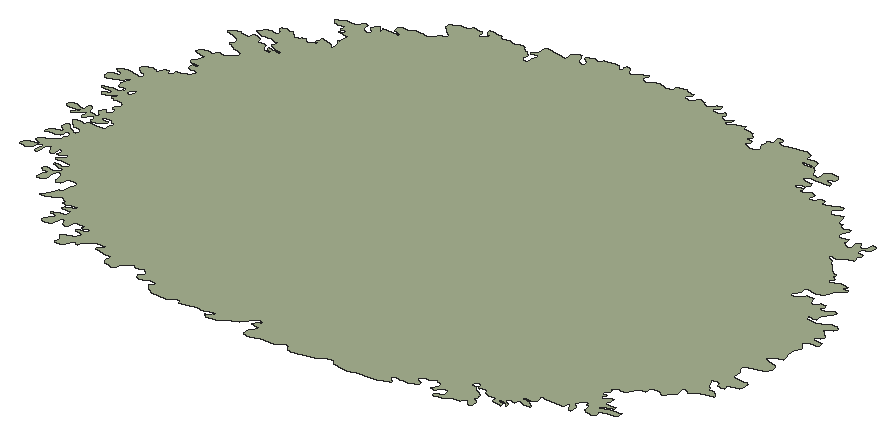
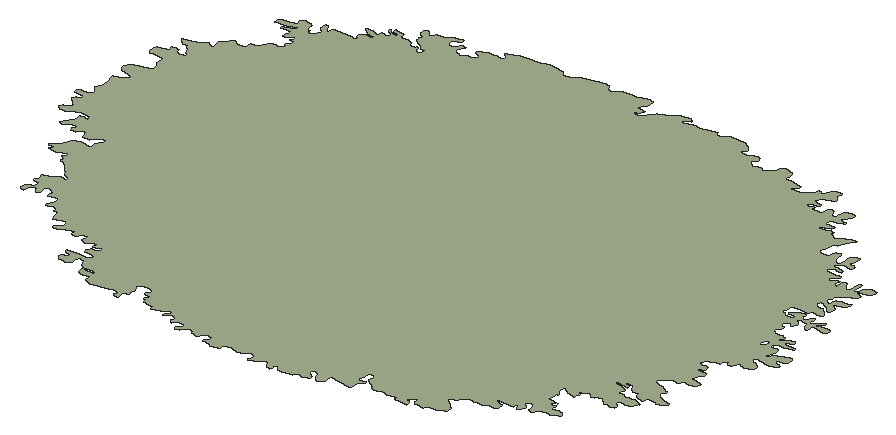
# SketchUp Ruby script. Lengths in inches.
U = 1.inch
M = Sketchup.active_model
def pt(a) = Geom::Point3d.new(a.map { |v| v * U })
def face(e, loops, mat)
  f = e.add_face(loops[0].map { |a| pt(a) })
  loops[1..].each { |l| e.add_face(l.map { |a| pt(a) }).erase! }
  f.material = f.back_material = mat if mat
  f
end
# faces: each face lists its corners as indices into pts; further lists are holes
def faces(e, pts, list, mat = nil) = list.each { |f| face(e, (f[0].is_a?(Array) ? f : [f]).map { |l| l.map { |i| pts[i] } }, mat) }
# xy, xz, yz: faces in a plane at the given z, y or x. An outline is a flat list of corners, or four numbers for a rectangle; further outlines are holes
def ring(l) = l.size == 4 ? [[l[0], l[1]], [l[2], l[1]], [l[2], l[3]], [l[0], l[3]]] : l.each_slice(2).to_a
def flat(e, list, mat, &to3) = list.each { |f| face(e, (f[0].is_a?(Array) ? f : [f]).map { |l| ring(l).map { |u, v| to3.(u, v) } }, mat) }
def xy(e, z, list, mat = nil) = flat(e, list, mat) { |x, y| [x, y, z] }
def xz(e, y, list, mat = nil) = flat(e, list, mat) { |x, z| [x, y, z] }
def yz(e, x, list, mat = nil) = flat(e, list, mat) { |y, z| [x, y, z] }
def lines(e, pts, list) = list.each { |a, b| e.add_line(pt(pts[a]), pt(pts[b])) }
# prism: a flat outline (further loops are holes) pulled along v
def prism(e, loops, v, mat = nil)
  f = face(e, loops, mat); d = Geom::Vector3d.new(v.map { |x| x * U })
  f.pushpull(f.normal.samedirection?(d) ? d.length : -d.length)
end
def box(e, o, s, mat = nil) = prism(e, [[o, [o[0] + s[0], o[1], o[2]], [o[0] + s[0], o[1] + s[1], o[2]], [o[0], o[1] + s[1], o[2]]]], [0, 0, s[2]], mat)
def at(x, y, z, deg = 0) = Geom::Transformation.translation(pt([x, y, z])) * Geom::Transformation.rotation(ORIGIN, Z_AXIS, deg.degrees)
def axes(o, x, y, z) = Geom::Transformation.new([*x, 0, *y, 0, *z, 0, *pt(o).to_a, 1])
def part(name) = M.definitions.add(name)
# library, detail: a bought-in or finely detailed component or shape, given as its bounding box
def library(name, o, s) = part(name).tap { |d| box(d.entities, o, s) }
def detail(e, o, s) = box(e.add_group.entities, o, s)
def put(e, d, t, mat = nil) = e.add_instance(d, t).tap { |i| i.material = mat if mat }
def group(e, t, mat = nil) = e.add_group.tap { |g| g.transformation = t; g.material = mat if mat }.entities
root = M.entities
M.materials.add("Boxwoodplan").color = [166, 177, 144]
xy(root,9.058,[[[163.417,67.129,163.306,67.133,163.211,67.159,163.155,67.215,163.153,67.317,163.179,67.382,163.243,67.445,163.292,67.509,163.35,67.606,163.164,67.635,163.074,67.644,163.094,67.732,163.18,67.79,163.211,67.8,163.206,67.846,163.117,67.877,163.001,67.837,162.904,67.706,162.761,67.551,162.6,67.464,162.495,67.441,162.434,67.416,162.418,67.373,162.274,67.281,162.08,67.251,161.991,67.26,161.911,67.306,161.911,67.328,161.956,67.359,162.047,67.437,162.115,67.483,162.026,67.498,161.913,67.48,161.793,67.436,161.697,67.445,161.6,67.454,161.503,67.447,161.376,67.403,161.176,67.356,161.087,67.349,161.049,67.443,161.041,67.465,160.974,67.473,160.885,67.454,160.716,67.336,160.516,67.328,160.286,67.353,160.119,67.446,159.978,67.61,160.161,67.702,160.061,67.756,159.925,67.772,159.799,67.749,159.727,67.697,159.646,67.672,159.53,67.738,159.488,67.806,159.576,67.847,159.602,67.907,159.607,67.957,159.566,68.009,159.494,68.085,159.408,68.117,159.321,68.064,159.255,68.038,159.199,68.08,159.182,68.103,159.158,68.121,159.129,68.111,159.049,68.058,158.978,68.01,158.902,67.923,158.89,67.79,158.819,67.749,158.769,67.723,158.709,67.725,158.61,67.746,158.523,67.793,158.479,67.861,158.471,67.951,158.48,68.018,158.493,68.04,158.474,68.08,158.26,68.1,158.328,68.135,158.302,68.136,158.209,68.13,158.039,68.146,157.962,68.173,157.945,68.206,157.96,68.224,158.085,68.314,158.083,68.371,157.998,68.393,157.839,68.39,157.708,68.319,157.611,68.233,157.536,68.199,157.489,68.172,157.488,68.154,157.524,68.101,157.508,68.046,157.438,68.081,157.374,68.121,157.313,68.072,157.291,68.017,157.259,67.904,157.212,67.855,157.139,67.822,157.048,67.816,156.978,67.841,156.959,67.874,156.966,67.892,156.987,67.932,157.009,67.991,156.978,68.048,156.877,68.149,156.991,68.229,157.052,68.269,157.132,68.285,157.199,68.315,157.254,68.37,157.339,68.476,157.267,68.503,157.1875,68.511,157.055,68.53,157.017,68.565,157.024,68.584,157.099,68.62,157.261,68.657,157.303,68.709,157.298,68.748,157.272,68.764,157.122,68.711,157.076,68.732,157.077,68.752,157.1,68.814,156.939,68.825,156.858,68.833,156.804,68.826,156.797,68.806,156.781,68.71,156.766,68.642,156.724,68.591,156.677,68.578,156.658,68.594,156.599,68.639,156.554,68.757,156.515,68.783,156.488,68.784,156.434,68.777,156.427,68.757,156.425,68.641,156.371,68.523,156.31,68.449,156.23,68.419,156.151,68.422,156.105,68.448,156.072,68.506,156.072,68.564,156.126,68.677,156.24,68.784,156.26,68.803,156.247,68.823,156.22,68.829,156.14,68.847,156.059,68.86,156.032,68.875,156.039,68.895,156.059,68.914,156.208,68.982,156.37,69.005,156.412,69.108,156.385,69.169,156.338,69.191,156.311,69.187,156.148,69.168,156.107,69.2,156.114,69.22,156.141,69.279,156.299,69.334,156.471,69.403,156.519,69.442,156.506,69.463,156.409,69.436,156.238,69.417,156.094,69.372,156.005,69.386,155.978,69.392,155.984,69.412,156.005,69.426,156.06,69.47,156.032,69.507,156.005,69.503,155.922,69.511,155.867,69.56,155.853,69.601,155.826,69.597,155.743,69.575,155.586,69.489,155.437,69.413,155.363,69.38,155.308,69.392,155.321,69.412,155.34,69.452,155.367,69.469,155.391,69.55,155.441,69.65,155.473,69.759,155.524,69.812,155.597,69.852,155.641,69.972,155.663,70.112,155.683,70.227,155.679,70.285,155.634,70.321,155.553,70.335,155.467,70.335,155.393,70.31,155.383,70.245,155.384,70.184,155.351,70.124,155.263,70.087,155.206,70.096,155.168,70.155,155.157,70.216,155.131,70.337,155.126,70.4,155.085,70.453,155.058,70.475,155.02,70.491,154.961,70.479,154.927,70.46,154.925,70.428,154.917,70.366,154.92,70.229,154.945,70.167,154.937,70.103,154.886,70.038,154.838,70.01,154.8,69.998,154.762,70.003,154.72,70.011,154.702,70.039,154.698,70.166,154.719,70.223,154.764,70.276,154.78,70.306,154.772,70.334,154.715,70.34,154.633,70.346,154.596,70.362,154.573,70.39,154.57,70.453,154.585,70.483,154.62,70.499,154.792,70.472,154.871,70.497,154.92,70.526,154.981,70.573,154.994,70.636,154.971,70.662,154.927,70.664,154.85,70.67,154.758,70.681,154.657,70.717,154.638,70.746,154.644,70.76,154.663,70.763,154.723,70.775,154.898,70.761,154.988,70.787,155,70.844,154.974,70.907,154.902,70.946,154.823,70.953,154.71,70.946,154.61,70.921,154.527,70.939,154.523,70.968,154.543,70.997,154.59,71.054,154.656,71.11,154.709,71.19,154.701,71.224,154.656,71.241,154.591,71.24,154.473,71.14,154.433,71.141,154.399,71.161,154.421,71.22,154.437,71.287,154.394,71.35,154.354,71.366,154.334,71.367,154.328,71.352,154.332,71.306,154.329,71.164,154.288,71.102,154.249,71.108,154.214,71.131,154.116,71.262,154.092,71.327,154.067,71.355,154.052,71.344,153.996,71.293,153.961,71.234,153.981,71.103,153.986,71.037,153.966,70.971,153.916,70.962,153.882,70.978,153.872,71.023,153.892,71.155,153.901,71.233,153.901,71.27,153.886,71.282,153.871,71.272,153.792,71.237,153.752,71.183,153.743,71.12,153.704,71.077,153.567,70.987,153.527,70.977,153.483,70.986,153.403,71.026,153.383,71.056,153.387,71.089,153.42,71.151,153.517,71.237,153.607,71.263,153.697,71.263,153.792,71.267,153.731,71.318,153.58,71.404,153.563,71.466,153.616,71.503,153.708,71.573,153.827,71.635,153.945,71.709,153.981,71.723,154.007,71.746,154.033,71.789,154.036,71.882,154.069,72.003,154.07,72.065,154.049,72.086,154.027,72.095,153.964,72.109,153.931,72.104,153.927,72.088,153.939,71.996,153.897,71.934,153.849,71.899,153.772,71.871,153.701,71.858,153.54,71.833,153.505,71.839,153.492,71.853,153.492,71.86,153.501,71.901,153.518,71.947,153.56,71.995,153.629,72.042,153.688,72.063,153.746,72.065,153.785,72.068,153.805,72.075,153.828,72.096,153.823,72.121,153.769,72.151,153.701,72.207,153.669,72.264,153.665,72.331,153.678,72.382,153.73,72.426,153.756,72.432,153.767,72.425,153.787,72.411,153.83,72.35,153.879,72.304,154.007,72.226,154.081,72.192,154.116,72.177,154.136,72.184,154.16,72.206,154.167,72.222,154.178,72.263,154.163,72.32,154.12,72.366,154.088,72.389,154.054,72.401,153.994,72.401,153.92,72.404,153.877,72.446,153.791,72.519,153.732,72.569,153.693,72.617,153.694,72.646,153.718,72.671,153.774,72.698,153.809,72.703,153.85,72.7,153.91,72.679,153.972,72.677,154.008,72.684,154.042,72.726,154.091,72.757,154.15,72.764,154.221,72.764,154.375,72.771,154.515,72.792,154.548,72.808,154.549,72.826,154.543,72.868,154.531,72.913,154.542,72.957,154.572,73.06,154.559,73.083,154.536,73.097,154.479,73.126,154.426,73.164,154.353,73.192,154.28,73.195,154.23,73.184,154.209,73.17,154.184,73.119,154.189,73.098,154.2,73.093,154.224,73.088,154.375,73.076,154.401,73.071,154.406,73.0625,154.397,73.046,154.357,73.007,154.312,72.964,154.247,72.928,154.185,72.884,154.113,72.849,154.076,72.852,154.056,72.863,154.031,72.9,154.024,72.995,154.007,73.02,154.025,73.034,154.031,73.077,154.025,73.088,154.014,73.088,153.999,73.087,153.973,73.083,153.941,73.076,153.923,73.065,153.842,72.97,153.81,72.915,153.779,72.892,153.756,72.895,153.73,72.916,153.721,72.932,153.715,72.973,153.744,73.057,153.749,73.102,153.74,73.13,153.72,73.137,153.682,73.128,153.662,73.114,153.616,73.064,153.494,72.957,153.458,72.932,153.432,72.927,153.395,72.935,153.383,72.951,153.474,73.057,153.537,73.102,153.551,73.129,153.55,73.145,153.541,73.152,153.53,73.148,153.515,73.143,153.484,73.131,153.4,73.108,153.233,73.089,153.16,73.096,153.112,73.121,153.09,73.149,153.089,73.165,153.106,73.217,153.154,73.264,153.214,73.281,153.285,73.284,153.359,73.266,153.487,73.223,153.573,73.197,153.584,73.201,153.584,73.22,153.575,73.239,153.55,73.287,153.549,73.342,153.556,73.407,153.568,73.437,153.585,73.45,153.634,73.413,153.673,73.363,153.7,73.317,153.71,73.255,153.722,73.204,153.737,73.176,153.76,73.175,153.895,73.157,153.968,73.144,154.003,73.14,154.021,73.154,154.036,73.202,153.981,73.244,153.922,73.309,153.905,73.335,153.905,73.352,153.939,73.46,153.969,73.483,153.996,73.489,154.011,73.477,154.02,73.459,154.049,73.414,154.06,73.39,154.072,73.391,154.093,73.404,154.173,73.482,154.19,73.528,154.191,73.579,154.177,73.611,154.156,73.623,154.093,73.646,154.053,73.666,154.045,73.687,154.061,73.736,154.117,73.773,154.151,73.795,154.164,73.816,154.172,73.869,154.17,73.916,154.075,73.992,153.931,74.014,153.869,74.031,153.834,74.013,153.806,74.014,153.737,74.031,153.718,74.058,153.727,74.082,153.853,74.185,153.847,74.217,153.825,74.233,153.78,74.225,153.751,74.216,153.625,74.154,153.585,74.107,153.536,74.063,153.467,74.049,153.439,74.05,153.392,74.102,153.42,74.126,153.4375,74.165,153.469,74.188,153.563,74.22,153.608,74.25,153.597,74.281,153.584,74.283,153.574,74.276,153.548,74.27,153.509,74.273,153.374,74.284,153.227,74.3125,153.203,74.327,153.209,74.347,153.234,74.375,153.447,74.435,153.51,74.434,153.571,74.419,153.631,74.391,153.658,74.393,153.664,74.403,153.713,74.48,153.737,74.495,153.743,74.515,153.743,74.583,153.732,74.593,153.719,74.591,153.661,74.591,153.604,74.585,153.557,74.568,153.533,74.576,153.512,74.596,153.487,74.63,153.467,74.718,153.478,74.806,153.508,74.848,153.514,74.88,153.527,74.923,153.564,74.944,153.56,74.99,153.538,75.026,153.449,75.003,153.431,74.969,153.432,74.95,153.435,74.886,153.355,74.839,153.214,74.745,153.058,74.7,152.974,74.725,152.932,74.778,152.923,74.904,153.051,74.99,153.134,75.003,153.177,75.027,153.201,75.061,153.2,75.081,153.114,75.112,153.041,75.138,152.979,75.194,153.014,75.249,153.09,75.278,153.186,75.312,153.251,75.311,153.43,75.267,153.522,75.246,153.607,75.25,153.658,75.269,153.664,75.289,153.648,75.355,153.587,75.407,153.542,75.415,153.43,75.485,153.383,75.527,153.369,75.564,153.362,75.617,153.362,75.644,153.375,75.659,153.417,75.695,153.468,75.709,153.582,75.741,153.613,75.751,153.653,75.75,153.703,75.746,153.716,75.733,153.731,75.703,153.745,75.689,153.755,75.689,153.783,75.692,153.799,75.704,153.82,75.754,153.848,75.787,153.864,75.81,153.867,75.835,153.883,75.86,153.903,75.872,153.951,75.884,153.99,75.877,154.011,75.833,154.015,75.781,154.032,75.755,154.053,75.754,154.095,75.796,154.12,75.838,154.134,75.942,154.15,75.968,154.182,75.975,154.214,75.974,154.233,75.963,154.254,75.94,154.286,75.94,154.339,75.961,154.383,76.007,154.397,76.032,154.386,76.046,154.446,76.043,154.475,76.046,154.491,76.066,154.496,76.114,154.53,76.155,154.564,76.2,154.51,76.243,154.443,76.272,154.406,76.271,154.373,76.261,154.331,76.249,154.289,76.255,154.267,76.271,154.246,76.295,154.223,76.397,154.236,76.423,154.241,76.439,154.251,76.443,154.356,76.463,154.402,76.472,154.42,76.483,154.41,76.486,154.324,76.514,154.258,76.526,154.23,76.519,154.195,76.52,154.159,76.52,154.123,76.532,154.085,76.582,154.067,76.611,154.067,76.642,154.082,76.663,154.111,76.678,154.142,76.697,154.15,76.725,154.18,76.782,154.207,76.836,154.213,76.89,154.206,76.917,154.166,76.928,154.088,76.954,153.915,77.001,153.879,77.018,153.862,77.042,153.898,77.097,153.942,77.131,153.988,77.159,154.043,77.178,154.095,77.1875,154.148,77.184,154.203,77.16,154.258,77.162,154.285,77.167,154.298,77.187,154.315,77.228,154.352,77.264,154.373,77.282,154.399,77.284,154.468,77.267,154.53,77.256,154.556,77.253,154.58,77.268,154.667,77.336,154.754,77.401,154.808,77.498,154.804,77.542,154.763,77.579,154.646,77.617,154.52,77.647,154.434,77.719,154.376,77.755,154.307,77.776,154.28,77.788,154.266,77.808,154.288,77.855,154.336,77.896,154.334,77.981,154.284,78.06,154.154,78.116,153.866,78.212,153.845,78.246,153.917,78.31,154.038,78.362,154.143,78.367,154.2,78.353,154.244,78.327,154.293,78.317,154.346,78.326,154.407,78.337,154.436,78.368,154.451,78.448,154.468,78.483,154.522,78.482,154.579,78.471,154.627,78.451,154.694,78.392,154.718,78.358,154.732,78.318,154.733,78.249,154.739,78.245,154.748,78.249,154.775,78.262,154.826,78.268,154.915,78.271,154.995,78.235,155.029,78.17,155.054,78.092,155.124,78.047,155.164,78.035,155.182,78.034,155.209,78.043,155.304,78.05,155.321,78.055,155.301,78.071,155.238,78.095,155.186,78.099,155.148,78.118,155.129,78.152,155.126,78.164,155.129,78.184,155.144,78.191,155.179,78.192,155.221,78.185,155.327,78.156,155.442,78.152,155.494,78.159,155.512,78.162,155.538,78.173,155.494,78.203,155.453,78.213,155.367,78.228,155.309,78.242,155.268,78.244,155.246,78.248,155.221,78.263,155.169,78.289,155.122,78.315,155.1,78.348,155.11,78.404,155.139,78.442,155.18,78.471,155.14,78.502,155.085,78.517,155.042,78.52,154.987,78.528,154.956,78.555,154.938,78.591,154.924,78.6,154.895,78.599,154.779,78.571,154.727,78.557,154.678,78.559,154.63,78.562,154.581,78.578,154.533,78.595,154.493,78.602,154.407,78.65,154.432,78.662,154.434,78.669,154.445,78.709,154.461,78.745,154.487,78.782,154.518,78.814,154.562,78.839,154.615,78.862,154.66,78.873,154.766,78.867,154.843,78.862,154.876,78.858,154.887,78.857,154.887,78.87,154.879,78.912,154.858,78.956,154.822,78.995,154.779,79.026,154.746,79.073,154.748,79.096,154.759,79.117,154.806,79.147,154.858,79.17,154.885,79.169,154.911,79.163,154.965,79.148,155.033,79.142,155.08,79.127,155.104,79.114,155.122,79.095,155.166,79.055,155.205,79.02,155.25,78.989,155.306,78.976,155.36,78.981,155.405,79.01,155.437,79.046,155.486,79.084,155.512,79.083,155.534,79.069,155.575,79.027,155.622,78.994,155.75,79.019,155.824,79.037,155.865,79.065,155.871,79.085,155.85,79.102,155.799,79.124,155.789,79.147,155.797,79.169,155.813,79.214,155.82,79.273,155.824,79.299,155.847,79.315,155.874,79.316,155.904,79.308,155.946,79.288,156.08,79.248,156.141,79.226,156.18,79.193,156.207,79.153,156.222,79.13,156.229,79.123,156.238,79.126,156.246,79.131,156.279,79.176,156.285,79.212,156.275,79.315,156.253,79.362,156.229,79.397,156.194,79.436,156.184,79.466,156.195,79.477,156.206,79.475,156.228,79.476,156.227,79.484,156.232,79.508,156.225,79.549,156.21,79.705,156.212,79.782,156.097,79.802,156,79.804,155.9375,79.8125,155.92,79.819,155.906,79.83,155.919,79.839,156.032,79.882,156.066,79.911,156.065,79.924,156.042,79.948,156.006,79.952,155.953,79.94,155.905,79.918,155.888,79.919,155.873,79.945,155.899,80.028,155.902,80.069,155.901,80.082,155.877,80.103,155.788,80.085,155.675,80.088,155.566,80.105,155.505,80.185,155.503,80.213,155.541,80.25,155.637,80.303,155.686,80.33,155.74,80.335,155.865,80.332,155.956,80.337,156.016,80.346,156.056,80.384,156.096,80.418,156.104,80.461,156.13,80.5,156.186,80.513,156.223,80.509,156.266,80.475,156.277,80.389,156.284,80.3,156.308,80.257,156.363,80.231,156.455,80.212,156.51,80.234,156.528,80.276,156.505,80.319,156.458,80.355,156.402,80.442,156.438,80.521,156.512,80.603,156.531,80.606,156.555,80.576,156.574,80.528,156.648,80.447,156.676,80.421,156.667,80.475,156.649,80.57,156.705,80.587,156.766,80.582,156.893,80.578,157.006,80.575,157.128,80.557,157.146,80.557,157.134,80.587,157.083,80.629,156.953,80.681,156.915,80.689,156.892,80.735,156.894,80.826,156.929,80.871,156.978,80.896,157.094,80.901,157.191,80.91,157.286,80.977,157.412,80.982,157.528,80.971,157.624,80.953,157.745,80.946,157.788,80.991,157.801,81.038,157.844,81.133,157.933,81.187,158.053,81.244,158.065,81.26,158.048,81.294,158.007,81.332,157.9,81.413,157.832,81.487,157.774,81.528,157.717,81.57,157.748,81.577,157.747,81.591,157.742,81.612,157.731,81.679,157.734,81.709,157.769,81.744,157.852,81.785,157.935,81.821,157.973,81.827,158.029,81.826,158.116,81.816,158.139,81.808,158.163,81.81,158.195,81.843,158.247,81.918,158.283,81.932,158.34,81.936,158.442,81.93,158.538,81.898,158.57,81.877,158.599,81.835,158.6,81.765,158.603,81.736,158.608,81.715,158.631,81.704,158.684,81.715,158.729,81.745,158.791,81.798,158.816,81.822,158.837,81.834,158.85,81.85,158.765,81.897,158.727,81.913,158.684,81.956,158.659,82.036,158.66,82.067,158.718,82.083,158.91,82.055,159.007,82.039,159.042,82.026,159.042,81.98,159.052,81.952,159.112,81.948,159.216,81.962,159.318,81.975,159.36,81.971,159.407,81.957,159.434,81.934,159.459,81.933,159.484,81.943,159.628,81.972,159.669,81.981,159.721,81.987,159.757,81.984,159.802,81.957,159.832,81.886,159.858,81.863,159.903,81.844,159.943,81.833,159.983,81.808,160.035,81.753,160.089,81.696,160.076,81.619,160.069,81.545,160.083,81.515,160.114,81.485,160.141,81.461,160.188,81.453,160.224,81.45,160.269,81.481,160.282,81.512,160.283,81.553,160.271,81.628,160.308,81.787,160.297,81.817,160.279,81.829,160.255,81.833,160.216,81.834,160.164,81.828,160.128,81.826,160.081,81.835,160.056,81.858,160.063,81.88,160.091,81.896,160.13,81.91,160.175,81.937,160.2,82.013,160.204,82.178,160.204,82.21,160.227,82.228,160.253,82.233,160.352,82.222,160.551,82.201,160.642,82.19,160.731,82.169,160.818,82.153,160.869,82.147,160.864,82.355,160.932,82.427,161.017,82.486,161.071,82.477,161.099,82.441,161.147,82.37,161.17,82.297,161.178,82.26,161.176,82.241,161.203,82.206,161.308,82.173,161.36,82.173,161.399,82.204,161.402,82.279,161.299,82.36,161.221,82.419,161.233,82.453,161.277,82.49,161.371,82.541,161.421,82.55,161.502,82.538,161.606,82.537,161.629,82.615,161.839,82.643,161.939,82.661,162.047,82.647,162.126,82.578,162.159,82.543,162.186,82.541,162.226,82.568,162.224,82.643,162.215,82.685,162.228,82.72,162.278,82.729,162.333,82.715,162.404,82.621,162.425,82.548,162.458,82.513,162.507,82.498,162.558,82.503,162.604,82.53,162.692,82.613,162.773,82.668,162.875,82.715,162.923,82.7,162.937,82.663,162.885,82.592,162.859,82.557,162.867,82.515,162.956,82.457,163.056,82.443,163.106,82.452,163.156,82.498,163.234,82.566,163.349,82.581,163.464,82.553,163.495,82.523,163.572,82.492,163.672,82.511,163.754,82.565,163.754,82.678,163.811,82.721,163.924,82.745,164.029,82.74,164.11,82.681,164.256,82.66,164.31,82.651,164.316,82.614,164.242,82.546,164.209,82.473,164.221,82.437,164.293,82.396,164.395,82.401,164.448,82.433,164.468,82.472,164.488,82.544,164.537,82.567,164.561,82.579,164.612,82.579,164.715,82.541,164.758,82.47,164.844,82.417,164.974,82.447,165.009,82.478,165.015,82.52,165.055,82.603,165.162,82.622,165.192,82.592,165.198,82.55,165.145,82.466,165.097,82.448,165.07,82.413,165.13,82.349,165.261,82.337,165.352,82.373,165.419,82.444,165.444,82.45,165.453,82.433,165.471,82.392,165.495,82.357,165.484,82.301,165.464,82.257,165.482,82.222,165.571,82.179,165.679,82.184,165.734,82.203,165.785,82.258,165.802,82.273,165.804,82.255,165.791,82.212,165.718,82.132,165.684,82.102,165.695,82.066,165.742,82.047,165.8,82.048,165.896,82.088,165.978,82.146,166.198,82.225,166.22,82.153,166.243,82.123,166.294,82.118,166.41,82.11,166.534,82.084,166.549,82.013,166.572,81.983,166.618,81.964,166.641,81.93,166.627,81.892,166.6,81.795,166.717,81.773,166.763,81.755,166.773,81.72,166.699,81.65,166.685,81.613,166.701,81.579,166.777,81.527,166.88,81.5,166.981,81.496,167.093,81.563,167.135,81.639,167.077,81.71,167.044,81.779,167.064,81.885,167.073,81.922,167.044,81.956,167.04,81.992,167.082,82.018,167.183,82.022,167.172,82.122,167.13,82.274,167.18,82.287,167.245,82.275,167.298,82.256,167.329,82.199,167.279,82.131,167.283,82.095,167.329,82.076,167.437,82.076,167.567,82.111,168.074,82.178,168.12,82.168,168.166,82.145,168.212,82.121,168.246,82.097,168.277,82.027,168.26,81.935,168.464,81.949,168.529,81.943,168.614,81.911,168.651,81.805,168.636,81.757,168.62,81.724,168.579,81.717,168.409,81.749,168.345,81.755,168.302,81.755,168.282,81.749,168.279,81.733,168.307,81.685,168.348,81.666,168.395,81.666,168.568,81.681,168.637,81.683,168.721,81.648,168.758,81.609,168.789,81.546,168.857,81.437,168.936,81.398,169.021,81.394,169.052,81.435,169.046,81.518,169.028,81.571,169.035,81.637,169.076,81.687,169.177,81.719,169.286,81.732,169.375,81.701,169.423,81.659,169.457,81.597,169.458,81.551,169.396,81.495,169.33,81.482,169.289,81.471,169.257,81.437,169.261,81.407,169.31,81.389,169.408,81.363,169.479,81.339,169.499,81.306,169.487,81.275,169.433,81.247,169.346,81.24,169.184,81.233,169.097,81.222,169.008,81.256,168.944,81.269,168.862,81.251,168.806,81.208,168.804,81.143,168.862,81.103,168.949,81.081,169.035,81.066,169.082,81.066,169.116,81.046,169.137,81.003,169.12,80.938,169.085,80.89,169.057,80.866,169.012,80.854,168.87,80.834,168.85,80.829,168.841,80.784,168.845,80.751,168.89,80.732,168.957,80.731,168.998,80.731,169.048,80.746,169.111,80.778,169.125,80.712,169.096,80.665,169.089,80.635,169.128,80.617,169.189,80.622,169.271,80.67,169.327,80.711,169.355,80.736,169.393,80.721,169.457,80.704,169.526,80.651,169.522,80.603,169.479,80.537,169.446,80.472,169.464,80.448,169.511,80.445,169.587,80.456,169.669,80.495,169.708,80.554,169.78,80.597,169.84,80.609,169.877,80.601,169.895,80.577,169.898,80.548,169.881,80.521,169.853,80.497,169.855,80.483,169.876,80.481,170.048,80.499,170.129,80.51,170.196,80.552,170.238,80.589,170.317,80.614,170.414,80.619,170.437,80.595,170.44,80.566,170.28,80.349,170.295,80.304,170.352,80.251,170.435,80.237,170.524,80.255,170.592,80.283,170.677,80.305,170.742,80.213,170.778,79.999,170.78,79.985,170.816,79.974,170.9,79.996,170.911,79.918,170.935,79.871,171.011,79.861,171.148,79.896,171.216,79.893,171.231,79.839,171.163,79.619,171.152,79.567,171.175,79.514,171.241,79.486,171.309,79.496,171.445,79.523,171.465,79.419,171.46,79.316,171.582,79.247,171.715,79.216,171.745,79.318,171.735,79.421,171.712,79.474,171.74,79.525,171.809,79.535,171.848,79.482,171.87,79.429,171.918,79.395,171.995,79.418,172.049,79.467,172.073,79.583,172.077,79.636,172.138,79.659,172.195,79.631,172.225,79.577,172.2,79.455,172.085,79.375,172.032,79.339,172.011,79.282,171.991,79.231,172.014,79.186,172.146,79.161,172.202,79.134,172.207,79.083,172.134,78.997,172.169,78.895,172.198,78.844,172.186,78.794,172.052,78.768,171.951,78.729,171.847,78.658,171.796,78.623,171.73,78.626,171.666,78.659,171.634,78.667,171.608,78.643,171.652,78.549,171.771,78.483,171.818,78.445,171.815,78.396,171.9,78.32,172.066,78.132,172.198,78.05,172.261,78.035,172.298,77.992,172.283,77.898,172.399,77.834,172.336,77.749,172.316,77.697,172.314,77.673,172.345,77.661,172.482,77.679,172.617,77.755,172.747,77.768,172.872,77.734,172.875,77.687,172.809,77.66,172.783,77.644,172.797,77.62,172.875,77.599,172.947,77.596,172.979,77.595,172.992,77.571,172.904,77.482,172.738,77.322,172.714,77.232,172.71,77.187,172.682,77.142,172.589,77.067,172.461,77.038,172.336,77.043,172.227,77.082,172.158,77.076,172.131,77.004,172.158,76.894,172.129,76.787,172.011,76.72,172.039,76.62,172.177,76.642,172.349,76.833,172.576,76.815,172.652,76.605,172.697,76.595,172.779,76.618,172.866,76.723,173.004,76.735,173.042,76.635,172.992,76.574,172.977,76.539,173.054,76.501,173.193,76.531,173.3125,76.598,173.359,76.614,173.449,76.592,173.427,76.477,173.316,76.384,173.251,76.289,173.259,76.113,173.245,76.078,173.152,76.056,173.02,76.087,173.045,75.981,173.176,75.941,173.322,75.936,173.471,75.965,173.708,76.087,173.844,76.099,173.936,76.008,173.903,75.905,173.763,75.849,173.716,75.825,173.6875,75.766,173.791,75.675,173.942,75.515,173.909,75.414,173.793,75.359,173.757,75.335,173.795,75.274,173.939,75.269,174.069,75.247,174.081,75.145,174.008,75.089,173.875,75.078,173.75,75.041,173.707,74.942,173.875,74.761,173.768,74.568,173.771,74.388,173.825,74.176,173.869,74.078,173.737,74.051,173.614,74.008,173.52,73.931,173.493,73.869,173.604,73.801,173.856,73.744,173.933,73.662,173.954,73.559,173.912,73.467,173.797,73.394,173.336,73.234,173.338,73.141,173.382,73.048,173.436,72.954,173.4375,72.863,173.432,72.803,173.429,72.773,173.455,72.719,173.576,72.676,173.701,72.672,173.827,72.682,173.869,72.68,173.927,72.633,173.938,72.453,173.911,72.395,173.802,72.347,173.675,72.33,173.634,72.331,173.588,72.281,173.63,72.191,173.617,72.163,173.532,72.144,173.491,72.145,173.421,72.17,173.389,72.26,173.319,72.292,173.196,72.297,173.154,72.291,173.138,72.233,173.214,72.156,173.301,71.992,173.329,71.969,173.355,71.918,173.373,71.888,173.454,71.877,173.534,71.86,173.619,71.792,173.682,71.71,173.679,71.681,173.595,71.656,173.346,71.616,173.151,71.488,173.078,71.469,172.983,71.544,172.943,71.553,172.879,71.52,172.882,71.435,172.938,71.27,172.896,71.264,172.863,71.219,172.814,71.18,172.76,71.066,172.721,71.019,172.687,71,172.651,71.013,172.529,71.1,172.466,71.115,172.423,71.116,172.378,71.098,172.315,71.063,172.285,70.991,172.295,70.938,172.277,70.874,172.115,70.852,172.063,70.81,172.031,70.759,171.984,70.718,171.972,70.655,171.941,70.609,171.907,70.583,171.87,70.573,171.801,70.564,171.703,70.575,171.643,70.55,171.581,70.502,171.551,70.457,171.626,70.419,171.653,70.376,171.617,70.32,171.562,70.284,171.541,70.225,171.54,70.209,171.539,70.194,171.558,70.186,171.63,70.18,171.656,70.182,171.676,70.182,171.68,70.166,171.642,70.097,171.623,70.049,171.62,70.02,171.661,70.018,171.8,70.094,171.869,70.11,171.95,70.107,171.934,70.004,171.916,69.89,171.916,69.843,171.939,69.82,171.979,69.818,172.043,69.845,172.124,69.846,172.183,69.832,172.223,69.827,172.229,69.798,172.189,69.76,172.11,69.73,172.044,69.722,171.961,69.696,171.922,69.658,171.905,69.602,171.909,69.587,171.949,69.586,172.031,69.611,172.189,69.673,172.343,69.703,172.469,69.705,172.521,69.685,172.496,69.611,172.475,69.569,172.414,69.518,172.261,69.492,172.122,69.491,172.061,69.482,172.03,69.427,172.056,69.308,172.041,69.264,171.96,69.243,171.824,69.255,171.766,69.261,171.722,69.314,171.713,69.426,171.713,69.468,171.701,69.496,171.692,69.511,171.672,69.512,171.614,69.525,171.609,69.581,171.611,69.595,171.607,69.61,171.588,69.614,171.508,69.617,171.451,69.591,171.406,69.536,171.369,69.499,171.344,69.44,171.355,69.391,171.411,69.354,171.486,69.254,171.482,69.155,171.473,69.115,171.466,69.088,171.435,69.066,171.415,69.067,171.394,69.098,171.365,69.157,171.3,69.258,171.259,69.298,171.245,69.312,171.234,69.299,171.227,69.271,171.224,69.227,171.205,69.173,171.199,69.16,171.169,69.144,171.086,69.137,170.945,69.139,170.659,69.14,170.601,69.162,170.514,69.173,170.495,69.163,170.489,69.133,170.539,69.074,170.564,68.976,170.558,68.936,170.526,68.896,170.502,68.889,170.442,68.88,170.339,68.88,170.241,68.884,170.193,68.853,170.248,68.829,170.349,68.814,170.457,68.78,170.532,68.726,170.613,68.654,170.595,68.629,170.534,68.614,170.433,68.621,170.396,68.63,170.345,68.65,170.297,68.684,170.247,68.708,170.212,68.63,170.202,68.558,170.162,68.545,170.106,68.558,170.061,68.589,170.048,68.6,170.03,68.608,170.018,68.59,169.984,68.513,169.986,68.485,170.019,68.448,170.111,68.416,170.15,68.383,170.163,68.34,170.161,68.326,170.142,68.323,170.099,68.36,170.019,68.409,169.926,68.427,169.869,68.429,169.857,68.415,169.878,68.39,169.992,68.347,170.029,68.335,170.052,68.292,170.048,68.264,170.047,68.251,170.004,68.249,169.891,68.26,169.786,68.295,169.751,68.325,169.742,68.371,169.741,68.441,169.69,68.461,169.631,68.442,169.531,68.449,169.432,68.467,169.405,68.489,169.38,68.526,169.384,68.568,169.39,68.583,169.352,68.591,169.258,68.616,169.201,68.619,169.166,68.606,169.154,68.577,169.134,68.571,169.107,68.597,169.104,68.612,169.134,68.635,169.15,68.646,169.142,68.671,169.055,68.729,169.018,68.752,168.999,68.756,168.958,68.736,168.918,68.716,168.898,68.71,168.887,68.681,168.91,68.59,169.005,68.587,169.044,68.582,169.074,68.541,169.067,68.513,169.061,68.499,169.069,68.471,169.18,68.434,169.268,68.396,169.329,68.338,169.346,68.3125,169.345,68.299,169.31,68.283,169.29,68.273,169.321,68.251,169.376,68.225,169.388,68.2,169.337,68.168,169.325,68.141,169.35,68.106,169.435,68.062,169.513,67.994,169.512,67.851,169.491,67.825,169.439,67.814,169.385,67.829,169.347,67.874,169.307,67.939,169.289,67.949,169.251,67.944,169.199,67.926,169.177,67.897,169.178,67.854,169.177,67.84,169.144,67.828,168.967,67.819,168.959,67.826,168.911,67.808,168.867,67.777,168.783,67.692,168.731,67.661,168.657,67.651,168.519,67.643,168.465,67.658,168.463,67.698,168.572,67.762,168.672,67.834,168.669,67.937,168.663,67.98,168.663,67.994,168.632,68.015,168.572,68.034,168.498,68.034,168.414,67.95,168.394,67.911,168.337,67.866,168.322,67.857,168.286,67.865,168.249,67.88,168.237,67.907,168.277,67.999,168.337,68.094,168.338,68.135,168.27,68.189,168.159,68.224,168.107,68.246,168.07,68.238,168.045,68.215,168.011,68.171,167.978,68.156,167.936,68.157,167.88,68.166,167.843,68.168,167.805,68.145,167.724,68.05,167.738,68.01,167.812,67.97,167.867,67.938,167.894,67.917,167.903,67.89,167.879,67.851,167.819,67.807,167.717,67.756,167.662,67.735,167.589,67.738,167.534,67.76,167.46,67.769,167.415,67.745,167.378,67.743,167.346,67.76,167.291,67.766,167.218,67.752,167.196,67.717,167.206,67.659,167.303,67.575,167.33,67.536,167.331,67.51,167.331,67.497,167.313,67.492,167.023,67.391,166.748,67.369,166.515,67.373,166.424,67.371,166.302,67.31,166.199,67.275,166.102,67.279,166.064,67.281,166.015,67.299,165.967,67.328,165.906,67.325,165.817,67.334,165.733,67.376,165.673,67.433,165.642,67.478,165.583,67.491,165.484,67.479,165.388,67.438,165.308,67.398,165.209,67.325,165.112,67.269,165.019,67.24,164.778,67.222,164.588,67.186,164.491,67.19,164.426,67.284,164.395,67.351,164.307,67.365,164.216,67.352,164.12,67.28,164.055,67.217,163.965,67.21,163.788,67.233,163.603,67.24,163.525,67.189],[153.925,74.415,153.967,74.419,153.987,74.422,154.013,74.431,154.025,74.474,154.026,74.513,154.033,74.597,154.025,74.631,154.013,74.643,154.013,74.658,153.97,74.635,153.914,74.612,153.894,74.606,153.878,74.59,153.857,74.557,153.847,74.52,153.849,74.476,153.868,74.437,153.887,74.421]]],"Boxwoodplan")
